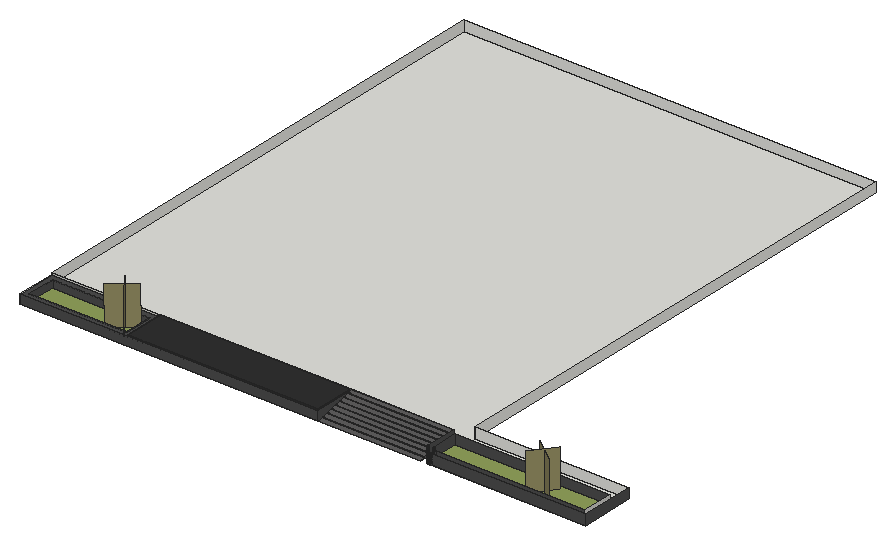
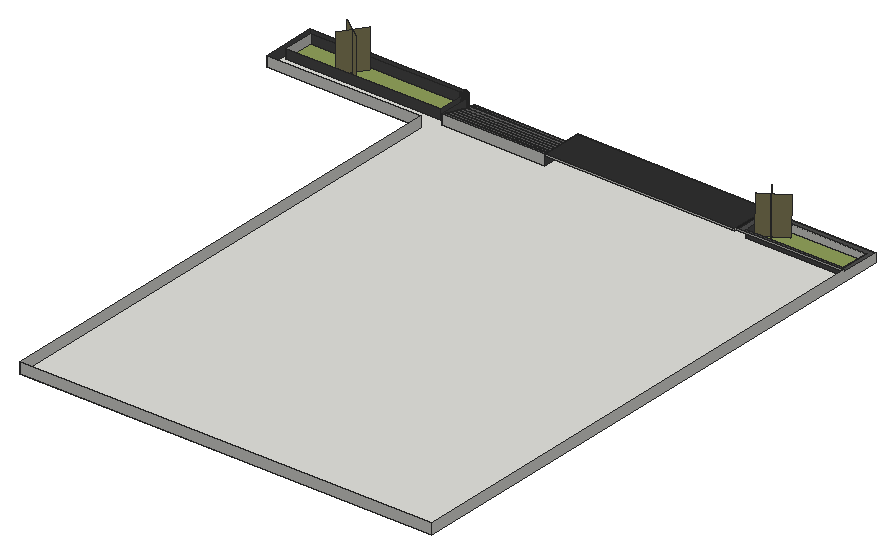
# SketchUp Ruby script. Lengths in inches.
U = 1.inch
M = Sketchup.active_model
def pt(a) = Geom::Point3d.new(a.map { |v| v * U })
def face(e, loops, mat)
  f = e.add_face(loops[0].map { |a| pt(a) })
  loops[1..].each { |l| e.add_face(l.map { |a| pt(a) }).erase! }
  f.material = f.back_material = mat if mat
  f
end
# faces: each face lists its corners as indices into pts; further lists are holes
def faces(e, pts, list, mat = nil) = list.each { |f| face(e, (f[0].is_a?(Array) ? f : [f]).map { |l| l.map { |i| pts[i] } }, mat) }
# xy, xz, yz: faces in a plane at the given z, y or x. An outline is a flat list of corners, or four numbers for a rectangle; further outlines are holes
def ring(l) = l.size == 4 ? [[l[0], l[1]], [l[2], l[1]], [l[2], l[3]], [l[0], l[3]]] : l.each_slice(2).to_a
def flat(e, list, mat, &to3) = list.each { |f| face(e, (f[0].is_a?(Array) ? f : [f]).map { |l| ring(l).map { |u, v| to3.(u, v) } }, mat) }
def xy(e, z, list, mat = nil) = flat(e, list, mat) { |x, y| [x, y, z] }
def xz(e, y, list, mat = nil) = flat(e, list, mat) { |x, z| [x, y, z] }
def yz(e, x, list, mat = nil) = flat(e, list, mat) { |y, z| [x, y, z] }
def lines(e, pts, list) = list.each { |a, b| e.add_line(pt(pts[a]), pt(pts[b])) }
# prism: a flat outline (further loops are holes) pulled along v
def prism(e, loops, v, mat = nil)
  f = face(e, loops, mat); d = Geom::Vector3d.new(v.map { |x| x * U })
  f.pushpull(f.normal.samedirection?(d) ? d.length : -d.length)
end
def box(e, o, s, mat = nil) = prism(e, [[o, [o[0] + s[0], o[1], o[2]], [o[0] + s[0], o[1] + s[1], o[2]], [o[0], o[1] + s[1], o[2]]]], [0, 0, s[2]], mat)
def at(x, y, z, deg = 0) = Geom::Transformation.translation(pt([x, y, z])) * Geom::Transformation.rotation(ORIGIN, Z_AXIS, deg.degrees)
def axes(o, x, y, z) = Geom::Transformation.new([*x, 0, *y, 0, *z, 0, *pt(o).to_a, 1])
def part(name) = M.definitions.add(name)
# library, detail: a bought-in or finely detailed component or shape, given as its bounding box
def library(name, o, s) = part(name).tap { |d| box(d.entities, o, s) }
def detail(e, o, s) = box(e.add_group.entities, o, s)
def put(e, d, t, mat = nil) = e.add_instance(d, t).tap { |i| i.material = mat if mat }
def group(e, t, mat = nil) = e.add_group.tap { |g| g.transformation = t; g.material = mat if mat }.entities
root = M.entities
M.materials.add("[Granite Dark Gray]1").color = [48, 48, 48]
M.materials.add("[Granite Dark Gray]2").color = [92, 91, 91]
M.materials.add("[Stone Coursed Rough]").color = [76, 76, 76]
M.materials.add("[Stone Sandstone Ashlar Light]").color = [206, 205, 201]
M.materials.add("[Vegetation Grass]").color = [144, 160, 91]
M.materials.add("tree").color = [143, 137, 96]
c1 = part("Component\#63")
g1 = group(c1.entities,at(22.42,-16.65,0.68))
p = [[0,0,71.01],[0,0,0],[30.99,41.73,0],[30.99,41.73,71.01]]
faces(g1,p,[[0,1,2,3]],"tree")
g2 = group(c1.entities,at(61.54,-11.49,0))
p = [[1.53,-1.19,70.99],[0,0,0],[-41.7,31,1.42],[-40.17,29.8,72.41]]
faces(g2,p,[[0,1,2,3]],"tree")
xy(root,-6,[[0,0,0,648,480,648,480,63,660,63,660,0,479.6875,0,479.53,0.01,479.37,0.02,479.22,0.03,478.9,0.05,478.75,0.07,478.59,0.08,478.43,0.1,478.28,0.125,478.12,0.15,477.97,0.17,477.8125,0.2,477.66,0.23,477.51,0.26,477.35,0.3,477.2,0.33,477.05,0.37,476.89,0.41,476.59,0.49,476.14,0.64,475.99,0.6875,475.85,0.74,475.7,0.8,475.55,0.85,475.41,0.91,475.26,0.97,475.12,1.04,474.98,1.1,474.83,1.17,474.27,1.45,474.14,1.53,474,1.61,473.86,1.6875,473.73,1.77,473.6,1.85,473.46,1.9375,473.33,2.02,473.07,2.2,472.95,2.29,472.82,2.38,472.69,2.48,472.57,2.58,472.45,2.67,472.33,2.77,472.09,2.98,471.97,3.08,471.85,3.1875,471.74,3.3,471.625,3.4,471.51,3.51,471.4,3.625,471.3,3.74,471.1875,3.85,471.08,3.97,470.98,4.09,470.77,4.33,470.67,4.45,470.58,4.57,470.48,4.69,470.38,4.82,470.29,4.95,470.2,5.07,470.02,5.33,469.9375,5.46,469.85,5.6,469.77,5.73,469.6875,5.86,469.61,6,469.53,6.14,469.45,6.27,469.17,6.83,469.1,6.98,469.04,7.12,468.97,7.26,468.91,7.41,468.85,7.55,468.8,7.7,468.74,7.85,468.6875,7.99,468.64,8.14,468.49,8.59,468.41,8.89,468.37,9.05,468.33,9.2,468.3,9.35,468.26,9.51,468.23,9.66,468.2,9.8125,468.17,9.97,468.15,10.12,468.125,10.28,468.1,10.43,468.08,10.59,468.07,10.75,468.05,10.9,468.03,11.22,468.02,11.37,468.01,11.53,468,11.6875,468,48,348,48,348,0]])
xy(root,-5,[[6,6,120,40],[479.76,6,654,6,654,42,474,42,474,11.76,474.01,11.6875,474.01,11.61,474.03,11.45,474.03,11.37,474.04,11.29,474.05,11.22,474.0625,11.14,474.07,11.0625,474.09,10.98,474.1,10.91,474.12,10.83,474.13,10.75,474.15,10.68,474.17,10.6,474.18,10.52,474.2,10.45,474.23,10.37,474.25,10.3,474.27,10.22,474.29,10.15,474.32,10.07,474.34,10,474.37,9.92,474.43,9.78,474.46,9.7,474.58,9.42,474.62,9.35,474.65,9.28,474.77,9.07,474.8,9,474.84,8.93,474.88,8.87,474.93,8.8,474.97,8.73,475.01,8.67,475.06,8.6,475.1,8.54,475.15,8.47,475.19,8.41,475.29,8.29,475.34,8.22,475.39,8.16,475.4375,8.1,475.49,8.04,475.54,7.99,475.59,7.93,475.65,7.87,475.7,7.8125,475.76,7.76,475.8125,7.7,475.87,7.65,475.93,7.59,475.99,7.54,476.04,7.49,476.1,7.4375,476.16,7.39,476.22,7.34,476.29,7.29,476.41,7.19,476.47,7.15,476.54,7.1,476.6,7.06,476.67,7.01,476.73,6.97,476.8,6.93,476.87,6.88,476.93,6.84,477,6.8,477.07,6.77,477.28,6.65,477.35,6.62,477.42,6.58,477.7,6.46,477.78,6.43,477.92,6.37,478,6.34,478.07,6.32,478.15,6.29,478.22,6.27,478.3,6.25,478.37,6.23,478.45,6.2,478.52,6.18,478.6,6.17,478.68,6.15,478.75,6.13,478.83,6.12,478.91,6.1,478.98,6.09,479.0625,6.07,479.14,6.0625,479.22,6.05,479.29,6.04,479.37,6.03,479.45,6.03,479.61,6.01,479.6875,6.01]],"[Vegetation Grass]")
xy(root,4,[[126,0,348,48]])
xy(root,4,[[[0,0,126,46],[6,6,120,40]]],"[Stone Coursed Rough]")
xz(root,0,[[0,-6,348,4],[479.6875,-6,479.84,6],[479.84,-6,480,6],[480,-6,660,6]],"[Stone Coursed Rough]")
xz(root,6,[[6,-5,120,4]])
xz(root,6,[[479.76,-5,479.84,6],[479.84,-5,479.92,6],[479.92,-5,480,6],[480,-5,654,6]],"[Stone Coursed Rough]")
xz(root,6.01,[[479.61,-5,479.6875,6]],"[Stone Coursed Rough]")
xz(root,6.03,[[479.37,-5,479.45,6]],"[Stone Coursed Rough]")
xz(root,40,[[6,-5,120,4]],"[Stone Coursed Rough]")
xz(root,42,[[474,-5,654,6]],"[Stone Coursed Rough]")
xz(root,46,[[0,4,126,6]],"[Stone Sandstone Ashlar Light]")
xz(root,48,[[348,-6,468,6],[126,4,348,6]])
xz(root,63,[[480,-6,660,6]])
xz(root,648,[[0,-6,480,6]])
yz(root,0,[[0,-6,0,4,46,4,46,6,648,6,648,-6]])
yz(root,6,[[6,-5,40,4]],"[Stone Coursed Rough]")
yz(root,120,[[6,-5,40,4]],"[Stone Coursed Rough]")
yz(root,126,[[46,4,48,6]])
yz(root,348,[[0,-6,48,4]],"[Stone Coursed Rough]")
yz(root,468,[[11.6875,-6,11.84,6],[11.84,-6,12,6],[12,-6,48,6]],"[Stone Coursed Rough]")
yz(root,474,[[11.76,-5,11.84,6],[11.84,-5,11.92,6],[11.92,-5,12,6],[12,-5,42,6]],"[Stone Coursed Rough]")
yz(root,474.01,[[11.61,-5,11.6875,6]],"[Stone Coursed Rough]")
yz(root,474.03,[[11.37,-5,11.45,6]],"[Stone Coursed Rough]")
yz(root,480,[[63,-6,648,6]])
yz(root,654,[[6,-5,42,6]],"[Stone Sandstone Ashlar Light]")
yz(root,660,[[0,-6,63,6]],"[Stone Coursed Rough]")
p = [[479.06,0.04,6],[478.9,0.05,6],[478.9,0.05,-6],[479.06,0.04,-6],[479.22,0.03,6],[479.22,0.03,-6],
  [479.37,0.02,6],[479.37,0.02,-6],[479.53,0.01,6],[479.53,0.01,-6],[479.6875,0,6],[479.6875,0,-6],
  [478.12,0.15,6],[477.97,0.17,6],[477.97,0.17,-6],[478.12,0.15,-6],[478.28,0.125,6],[478.28,0.125,-6],
  [478.43,0.1,6],[478.43,0.1,-6],[478.59,0.08,6],[478.59,0.08,-6],[478.75,0.07,6],[478.75,0.07,-6],
  [477.66,0.23,6],[477.51,0.26,6],[477.51,0.26,-6],[477.66,0.23,-6],[477.8125,0.2,6],[477.8125,0.2,-6],
  [477.2,0.33,6],[477.05,0.37,6],[477.05,0.37,-6],[477.2,0.33,-6],[477.35,0.3,6],[477.35,0.3,-6],
  [476.89,0.41,6],[476.74,0.45,6],[476.74,0.45,-6],[476.89,0.41,-6],[476.44,0.54,6],[476.29,0.59,6],
  [476.29,0.59,-6],[476.44,0.54,-6],[476.59,0.49,6],[476.59,0.49,-6],[476.14,0.64,6],[475.99,0.6875,6],
  [475.99,0.6875,-6],[476.14,0.64,-6],[475.85,0.74,6],[475.7,0.8,6],[475.7,0.8,-6],[475.85,0.74,-6],
  [475.55,0.85,6],[475.55,0.85,-6],[475.41,0.91,6],[475.26,0.97,6],[475.26,0.97,-6],[475.41,0.91,-6],
  [475.12,1.04,6],[474.98,1.1,6],[474.98,1.1,-6],[475.12,1.04,-6],[474.83,1.17,6],[474.83,1.17,-6],
  [474.69,1.24,6],[474.55,1.31,6],[474.55,1.31,-6],[474.69,1.24,-6],[474.41,1.38,6],[474.41,1.38,-6],
  [474.27,1.45,6],[474.27,1.45,-6],[474.14,1.53,6],[474,1.61,6],[474,1.61,-6],[474.14,1.53,-6],
  [473.86,1.6875,6],[473.86,1.6875,-6],[473.73,1.77,6],[473.73,1.77,-6],[473.6,1.85,6],[473.6,1.85,-6],
  [473.46,1.9375,6],[473.33,2.02,6],[473.33,2.02,-6],[473.46,1.9375,-6],[473.2,2.11,6],[473.2,2.11,-6],
  [473.07,2.2,6],[473.07,2.2,-6],[472.95,2.29,6],[472.95,2.29,-6],[472.82,2.38,6],[472.82,2.38,-6],
  [472.69,2.48,6],[472.69,2.48,-6],[472.57,2.58,6],[472.57,2.58,-6],[472.45,2.67,6],[472.45,2.67,-6],
  [472.33,2.77,6],[472.33,2.77,-6],[472.21,2.875,6],[472.21,2.875,-6],[472.09,2.98,6],[472.09,2.98,-6],
  [471.97,3.08,6],[471.97,3.08,-6],[471.85,3.1875,6],[471.85,3.1875,-6],[471.74,3.3,6],[471.74,3.3,-6],
  [471.625,3.4,6],[471.625,3.4,-6],[471.51,3.51,6],[471.51,3.51,-6],[471.4,3.625,6],[471.4,3.625,-6],
  [471.3,3.74,6],[471.3,3.74,-6],[471.1875,3.85,6],[471.1875,3.85,-6],[471.08,3.97,6],[471.08,3.97,-6],
  [470.98,4.09,6],[470.98,4.09,-6],[470.875,4.21,6],[470.875,4.21,-6],[470.77,4.33,6],[470.77,4.33,-6],
  [470.67,4.45,6],[470.67,4.45,-6],[470.58,4.57,6],[470.58,4.57,-6],[470.48,4.69,6],[470.48,4.69,-6],
  [470.38,4.82,6],[470.38,4.82,-6],[470.29,4.95,6],[470.29,4.95,-6],[470.2,5.07,6],[470.2,5.07,-6],
  [470.11,5.2,6],[470.11,5.2,-6],[470.02,5.33,6],[470.02,5.33,-6],[469.9375,5.46,6],[469.9375,5.46,-6],
  [469.85,5.6,6],[469.85,5.6,-6],[469.77,5.73,6],[469.77,5.73,-6],[469.6875,5.86,6],[469.6875,5.86,-6],
  [469.61,6,6],[469.61,6,-6],[469.53,6.14,6],[469.53,6.14,-6],[469.45,6.27,6],[469.45,6.27,-6],
  [469.38,6.41,6],[469.38,6.41,-6],[469.31,6.55,6],[469.31,6.55,-6],[469.24,6.69,6],[469.24,6.69,-6],
  [469.17,6.83,6],[469.17,6.83,-6],[469.1,6.98,6],[469.1,6.98,-6],[469.04,7.12,6],[469.04,7.12,-6],
  [468.97,7.26,6],[468.97,7.26,-6],[468.91,7.41,6],[468.91,7.41,-6],[468.85,7.55,6],[468.85,7.55,-6],
  [468.8,7.7,6],[468.8,7.7,-6],[468.74,7.85,6],[468.74,7.85,-6],[468.6875,7.99,6],[468.6875,7.99,-6],
  [468.64,8.14,6],[468.64,8.14,-6],[468.59,8.29,6],[468.59,8.29,-6],[468.54,8.44,6],[468.54,8.44,-6],
  [468.49,8.59,6],[468.49,8.59,-6],[468.45,8.74,6],[468.45,8.74,-6],[468.41,8.89,6],[468.41,8.89,-6],
  [468.37,9.05,6],[468.37,9.05,-6],[468.33,9.2,6],[468.33,9.2,-6],[468.3,9.35,6],[468.3,9.35,-6],
  [468.26,9.51,6],[468.26,9.51,-6],[468.23,9.66,6],[468.23,9.66,-6],[468.2,9.8125,6],[468.2,9.8125,-6],
  [468.17,9.97,6],[468.17,9.97,-6],[468.15,10.12,6],[468.15,10.12,-6],[468.125,10.28,6],[468.125,10.28,-6],
  [468.1,10.43,6],[468.1,10.43,-6],[468.08,10.59,6],[468.08,10.59,-6],[468.07,10.75,6],[468.07,10.75,-6],
  [468.05,10.9,6],[468.05,10.9,-6],[468.04,11.06,6],[468.04,11.06,-6],[468.03,11.22,6],[468.03,11.22,-6],
  [468.02,11.37,6],[468.02,11.37,-6],[468.01,11.53,6],[468.01,11.53,-6],[468,11.6875,6],[468,11.6875,-6],
  [479.22,6.05,6],[479.29,6.04,6],[479.29,6.04,-5],[479.22,6.05,-5],[479.37,6.03,6],[479.37,6.03,-5],
  [479.45,6.03,6],[479.53,6.02,6],[479.53,6.02,-5],[479.45,6.03,-5],[479.61,6.01,6],[479.61,6.01,-5],
  [479.6875,6.01,6],[479.76,6,6],[479.76,6,-5],[479.6875,6.01,-5],[478.6,6.17,6],[478.68,6.15,6],
  [478.68,6.15,-5],[478.6,6.17,-5],[478.75,6.13,6],[478.75,6.13,-5],[478.83,6.12,6],[478.83,6.12,-5],
  [478.91,6.1,6],[478.91,6.1,-5],[478.98,6.09,6],[478.98,6.09,-5],[479.0625,6.07,6],[479.0625,6.07,-5],
  [479.14,6.0625,6],[479.14,6.0625,-5],[478.22,6.27,6],[478.3,6.25,6],[478.3,6.25,-5],[478.22,6.27,-5],
  [478.37,6.23,6],[478.37,6.23,-5],[478.45,6.2,6],[478.45,6.2,-5],[478.52,6.18,6],[478.52,6.18,-5],
  [477.92,6.37,6],[478,6.34,6],[478,6.34,-5],[477.92,6.37,-5],[478.07,6.32,6],[478.07,6.32,-5],
  [478.15,6.29,6],[478.15,6.29,-5],[477.7,6.46,6],[477.78,6.43,6],[477.78,6.43,-5],[477.7,6.46,-5],
  [477.85,6.4,6],[477.85,6.4,-5],[477.49,6.55,6],[477.56,6.52,6],[477.56,6.52,-5],[477.49,6.55,-5],
  [477.63,6.49,6],[477.63,6.49,-5],[477.28,6.65,6],[477.35,6.62,6],[477.35,6.62,-5],[477.28,6.65,-5],
  [477.42,6.58,6],[477.42,6.58,-5],[477.07,6.77,6],[477.14,6.73,6],[477.14,6.73,-5],[477.07,6.77,-5],
  [477.21,6.69,6],[477.21,6.69,-5],[476.87,6.88,6],[476.93,6.84,6],[476.93,6.84,-5],[476.87,6.88,-5],
  [477,6.8,6],[477,6.8,-5],[476.73,6.97,6],[476.8,6.93,6],[476.8,6.93,-5],[476.73,6.97,-5],
  [476.6,7.06,6],[476.67,7.01,6],[476.67,7.01,-5],[476.6,7.06,-5],[476.41,7.19,6],[476.47,7.15,6],
  [476.47,7.15,-5],[476.41,7.19,-5],[476.54,7.1,6],[476.54,7.1,-5],[476.29,7.29,6],[476.35,7.24,6],
  [476.35,7.24,-5],[476.29,7.29,-5],[476.16,7.39,6],[476.22,7.34,6],[476.22,7.34,-5],[476.16,7.39,-5],
  [476.04,7.49,6],[476.1,7.4375,6],[476.1,7.4375,-5],[476.04,7.49,-5],[475.93,7.59,6],[475.99,7.54,6],
  [475.99,7.54,-5],[475.93,7.59,-5],[475.8125,7.7,6],[475.87,7.65,6],[475.87,7.65,-5],[475.8125,7.7,-5],
  [475.76,7.76,6],[475.76,7.76,-5],[475.65,7.87,6],[475.7,7.8125,6],[475.7,7.8125,-5],[475.65,7.87,-5],
  [475.54,7.99,6],[475.59,7.93,6],[475.59,7.93,-5],[475.54,7.99,-5],[475.4375,8.1,6],[475.49,8.04,6],
  [475.49,8.04,-5],[475.4375,8.1,-5],[475.39,8.16,6],[475.39,8.16,-5],[475.29,8.29,6],[475.34,8.22,6],
  [475.34,8.22,-5],[475.29,8.29,-5],[475.19,8.41,6],[475.24,8.35,6],[475.24,8.35,-5],[475.19,8.41,-5],
  [475.15,8.47,6],[475.15,8.47,-5],[475.06,8.6,6],[475.1,8.54,6],[475.1,8.54,-5],[475.06,8.6,-5],
  [475.01,8.67,6],[475.01,8.67,-5],[474.93,8.8,6],[474.97,8.73,6],[474.97,8.73,-5],[474.93,8.8,-5],
  [474.88,8.87,6],[474.88,8.87,-5],[474.8,9,6],[474.84,8.93,6],[474.84,8.93,-5],[474.8,9,-5],
  [474.77,9.07,6],[474.77,9.07,-5],[474.69,9.21,6],[474.73,9.14,6],[474.73,9.14,-5],[474.69,9.21,-5],
  [474.65,9.28,6],[474.65,9.28,-5],[474.58,9.42,6],[474.62,9.35,6],[474.62,9.35,-5],[474.58,9.42,-5],
  [474.55,9.49,6],[474.55,9.49,-5],[474.52,9.56,6],[474.52,9.56,-5],[474.46,9.7,6],[474.49,9.63,6],
  [474.49,9.63,-5],[474.46,9.7,-5],[474.43,9.78,6],[474.43,9.78,-5],[474.37,9.92,6],[474.4,9.85,6],
  [474.4,9.85,-5],[474.37,9.92,-5],[474.34,10,6],[474.34,10,-5],[474.32,10.07,6],[474.32,10.07,-5],
  [474.27,10.22,6],[474.29,10.15,6],[474.29,10.15,-5],[474.27,10.22,-5],[474.25,10.3,6],[474.25,10.3,-5],
  [474.23,10.37,6],[474.23,10.37,-5],[474.18,10.52,6],[474.2,10.45,6],[474.2,10.45,-5],[474.18,10.52,-5],
  [474.17,10.6,6],[474.17,10.6,-5],[474.15,10.68,6],[474.15,10.68,-5],[474.13,10.75,6],[474.13,10.75,-5],
  [474.1,10.91,6],[474.12,10.83,6],[474.12,10.83,-5],[474.1,10.91,-5],[474.09,10.98,6],[474.09,10.98,-5],
  [474.07,11.0625,6],[474.07,11.0625,-5],[474.05,11.22,6],[474.0625,11.14,6],[474.0625,11.14,-5],[474.05,11.22,-5],
  [474.04,11.29,6],[474.04,11.29,-5],[474.03,11.37,6],[474.03,11.37,-5],[474.01,11.61,6],[474.02,11.53,6],
  [474.02,11.53,-5],[474.01,11.61,-5],[474.03,11.45,6],[474.03,11.45,-5],[474,11.76,6],[474.01,11.6875,6],
  [474.01,11.6875,-5],[474,11.76,-5]]
faces(root,p,[[0,1,2,3],[4,0,3,5],[6,4,5,7],[8,6,7,9],[10,8,9,11],[12,13,14,15],[16,12,15,17],[18,16,17,19],
  [20,18,19,21],[22,20,21,23],[1,22,23,2],[24,25,26,27],[28,24,27,29],[13,28,29,14],[30,31,32,33],[34,30,33,35],
  [25,34,35,26],[36,37,38,39],[31,36,39,32],[40,41,42,43],[44,40,43,45],[37,44,45,38],[46,47,48,49],[41,46,49,42],
  [50,51,52,53],[47,50,53,48],[51,54,55,52],[56,57,58,59],[54,56,59,55],[60,61,62,63],[57,60,63,58],[61,64,65,62],
  [66,67,68,69],[64,66,69,65],[67,70,71,68],[70,72,73,71],[74,75,76,77],[72,74,77,73],[75,78,79,76],[78,80,81,79],
  [80,82,83,81],[84,85,86,87],[82,84,87,83],[85,88,89,86],[88,90,91,89],[90,92,93,91],[92,94,95,93],[94,96,97,95],
  [96,98,99,97],[98,100,101,99],[100,102,103,101],[102,104,105,103],[104,106,107,105],[106,108,109,107],[108,110,111,109],[110,112,113,111],
  [112,114,115,113],[114,116,117,115],[116,118,119,117],[118,120,121,119],[120,122,123,121],[122,124,125,123],[124,126,127,125],[126,128,129,127],
  [128,130,131,129],[130,132,133,131],[132,134,135,133],[134,136,137,135],[136,138,139,137],[138,140,141,139],[140,142,143,141],[142,144,145,143],
  [144,146,147,145],[146,148,149,147],[148,150,151,149],[150,152,153,151],[152,154,155,153],[154,156,157,155],[156,158,159,157],[158,160,161,159],
  [160,162,163,161],[162,164,165,163],[164,166,167,165],[166,168,169,167],[168,170,171,169],[170,172,173,171],[172,174,175,173],[174,176,177,175],
  [176,178,179,177],[178,180,181,179],[180,182,183,181],[182,184,185,183],[184,186,187,185],[186,188,189,187],[188,190,191,189],[190,192,193,191],
  [192,194,195,193],[194,196,197,195],[196,198,199,197],[198,200,201,199],[200,202,203,201],[202,204,205,203],[204,206,207,205],[206,208,209,207],
  [208,210,211,209],[210,212,213,211],[212,214,215,213],[214,216,217,215],[216,218,219,217],[218,220,221,219],[220,222,223,221],[222,224,225,223],
  [224,226,227,225],[226,228,229,227],[228,230,231,229],[230,232,233,231],[234,235,236,237],[235,238,239,236],[240,241,242,243],[241,244,245,242],
  [246,247,248,249],[250,251,252,253],[251,254,255,252],[254,256,257,255],[256,258,259,257],[258,260,261,259],[260,262,263,261],[262,264,265,263],
  [264,234,237,265],[266,267,268,269],[267,270,271,268],[270,272,273,271],[272,274,275,273],[274,250,253,275],[276,277,278,279],[277,280,281,278],
  [280,282,283,281],[282,266,269,283],[284,285,286,287],[285,288,289,286],[288,276,279,289],[290,291,292,293],[291,294,295,292],[294,284,287,295],
  [296,297,298,299],[297,300,301,298],[300,290,293,301],[302,303,304,305],[303,306,307,304],[306,296,299,307],[308,309,310,311],[309,312,313,310],
  [312,302,305,313],[314,315,316,317],[315,308,311,316],[318,319,320,321],[319,314,317,320],[322,323,324,325],[323,326,327,324],[326,318,321,327],
  [328,329,330,331],[329,322,325,330],[332,333,334,335],[333,328,331,334],[336,337,338,339],[337,332,335,338],[340,341,342,343],[341,336,339,342],
  [344,345,346,347],[345,340,343,346],[348,344,347,349],[350,351,352,353],[351,348,349,352],[354,355,356,357],[355,350,353,356],[358,359,360,361],
  [359,354,357,360],[362,358,361,363],[364,365,366,367],[365,362,363,366],[368,369,370,371],[369,364,367,370],[372,368,371,373],[374,375,376,377],
  [375,372,373,376],[378,374,377,379],[380,381,382,383],[381,378,379,382],[384,380,383,385],[386,387,388,389],[387,384,385,388],[390,386,389,391],
  [392,393,394,395],[393,390,391,394],[396,392,395,397],[398,399,400,401],[399,396,397,400],[402,398,401,403],[404,402,403,405],[406,407,408,409],
  [407,404,405,408],[410,406,409,411],[412,413,414,415],[413,410,411,414],[416,412,415,417],[418,416,417,419],[420,421,422,423],[421,418,419,422],
  [424,420,423,425],[426,424,425,427],[428,429,430,431],[429,426,427,430],[432,428,431,433],[434,432,433,435],[436,434,435,437],[438,439,440,441],
  [439,436,437,440],[442,438,441,443],[444,442,443,445],[446,447,448,449],[447,444,445,448],[450,446,449,451],[452,450,451,453],[454,455,456,457],
  [455,458,459,456],[460,461,462,463]],"[Stone Coursed Rough]")
g3 = group(root,at(348,0,-6),"[Granite Dark Gray]2")
prism(g3,[[[0,42.5,10.625],[0,48,12],[0,48,0],[0,0,0],[0,5.5,1.375],[0,5.5,1.125],[0,6,1.24],[0,6,1.5],[0,12,3],[0,12,2.75],[0,12.5,2.87],[0,12.5,3.125],[0,18,4.5],[0,18,4.25],[0,18.5,4.37],[0,18.5,4.625],[0,24,6],[0,24,5.75],[0,24.5,5.87],[0,24.5,6.125],[0,30,7.5],[0,30,7.25],[0,30.5,7.37],[0,30.5,7.625],[0,36,9],[0,36,8.75],[0,36.5,8.87],[0,36.5,9.125],[0,42,10.5],[0,42,10.25],[0,42.5,10.37]]],[120,0,0])
put(root,c1,axes([567.51,20.64,-5],[0.63,0,0],[0,0.63,0],[0,0,0.63]))
put(root,c1,axes([127.42,20.64,-5],[-0.63,0,0],[0,0.63,0],[0,0,0.63]))
g4 = group(root,at(126,0,4),"[Granite Dark Gray]1")
prism(g4,[[[222,48,0],[222,0,0],[0,0,0],[0,46,0],[0,48,0]]],[0,0,2])
